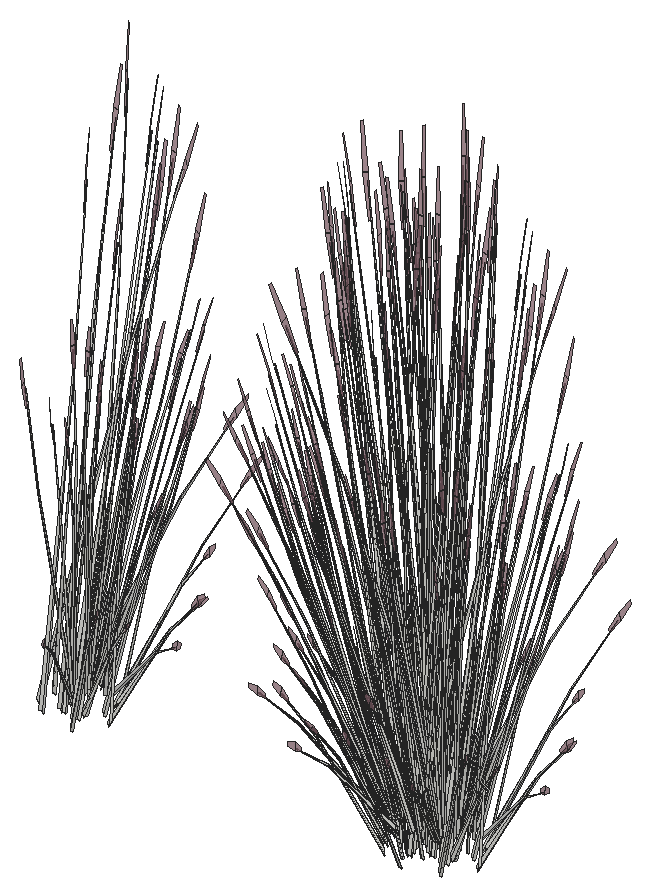
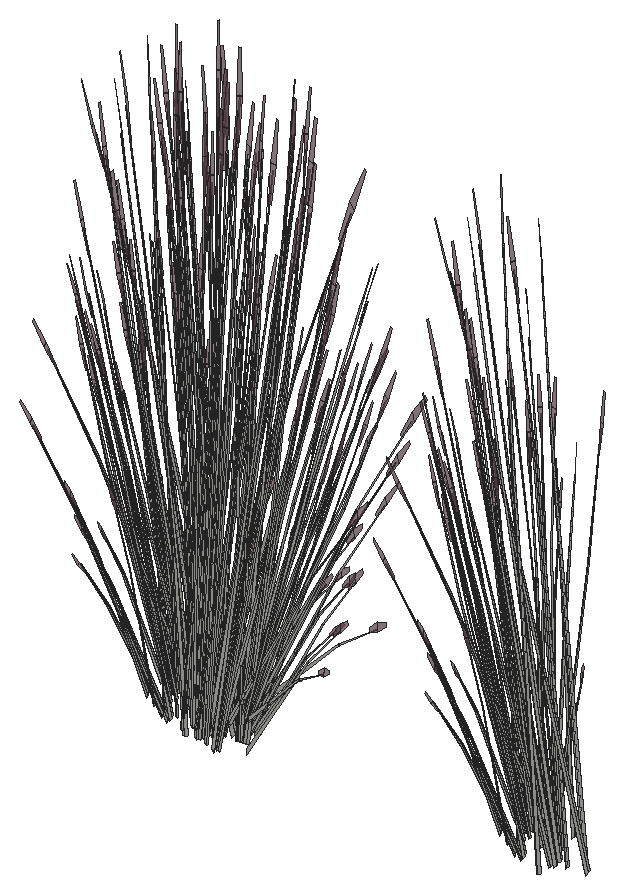
# SketchUp Ruby script. Lengths in inches.
U = 1.inch
M = Sketchup.active_model
def pt(a) = Geom::Point3d.new(a.map { |v| v * U })
def face(e, loops, mat)
  f = e.add_face(loops[0].map { |a| pt(a) })
  loops[1..].each { |l| e.add_face(l.map { |a| pt(a) }).erase! }
  f.material = f.back_material = mat if mat
  f
end
# faces: each face lists its corners as indices into pts; further lists are holes
def faces(e, pts, list, mat = nil) = list.each { |f| face(e, (f[0].is_a?(Array) ? f : [f]).map { |l| l.map { |i| pts[i] } }, mat) }
# xy, xz, yz: faces in a plane at the given z, y or x. An outline is a flat list of corners, or four numbers for a rectangle; further outlines are holes
def ring(l) = l.size == 4 ? [[l[0], l[1]], [l[2], l[1]], [l[2], l[3]], [l[0], l[3]]] : l.each_slice(2).to_a
def flat(e, list, mat, &to3) = list.each { |f| face(e, (f[0].is_a?(Array) ? f : [f]).map { |l| ring(l).map { |u, v| to3.(u, v) } }, mat) }
def xy(e, z, list, mat = nil) = flat(e, list, mat) { |x, y| [x, y, z] }
def xz(e, y, list, mat = nil) = flat(e, list, mat) { |x, z| [x, y, z] }
def yz(e, x, list, mat = nil) = flat(e, list, mat) { |y, z| [x, y, z] }
def lines(e, pts, list) = list.each { |a, b| e.add_line(pt(pts[a]), pt(pts[b])) }
# prism: a flat outline (further loops are holes) pulled along v
def prism(e, loops, v, mat = nil)
  f = face(e, loops, mat); d = Geom::Vector3d.new(v.map { |x| x * U })
  f.pushpull(f.normal.samedirection?(d) ? d.length : -d.length)
end
def box(e, o, s, mat = nil) = prism(e, [[o, [o[0] + s[0], o[1], o[2]], [o[0] + s[0], o[1] + s[1], o[2]], [o[0], o[1] + s[1], o[2]]]], [0, 0, s[2]], mat)
def at(x, y, z, deg = 0) = Geom::Transformation.translation(pt([x, y, z])) * Geom::Transformation.rotation(ORIGIN, Z_AXIS, deg.degrees)
def axes(o, x, y, z) = Geom::Transformation.new([*x, 0, *y, 0, *z, 0, *pt(o).to_a, 1])
def part(name) = M.definitions.add(name)
# library, detail: a bought-in or finely detailed component or shape, given as its bounding box
def library(name, o, s) = part(name).tap { |d| box(d.entities, o, s) }
def detail(e, o, s) = box(e.add_group.entities, o, s)
def put(e, d, t, mat = nil) = e.add_instance(d, t).tap { |i| i.material = mat if mat }
def group(e, t, mat = nil) = e.add_group.tap { |g| g.transformation = t; g.material = mat if mat }.entities
root = M.entities
M.materials.add("LightPink_Translucent").color = [144, 107, 117]
M.materials["LightPink_Translucent"].alpha = 0.75
c1 = part("blade")
p = [[2.15,0.21,22],[0,0.17,0],[0.09,0.45,0],[2.18,0.31,22],[2.29,0.31,22],[0.38,0.45,0],
  [2.48,0.24,33],[2.49,0.24,33],[2.48,0.22,33]]
faces(c1.entities,p,[[0,1,2,3],[4,5,2,3],[6,3,4,7],[8,0,3,6]])
c2 = part("seeds")
p = [[0.3,-0.1,1.38],[-0.01,-0.03,1.59],[-0.01,-0.03,0.03],[0.14,-0.07,-0.07],[0.29,-0.03,3],[0.15,0.01,3.11]]
faces(c2.entities,p,[[0,1,2,3],[1,0,4,5]],"LightPink_Translucent")
c3 = part("blade with seeds")
put(c3.entities,c1,at(0,0,0))
put(c3.entities,c2,axes([2.4,0.25,30.99],[1.5799,-0.05474,1.17369],[-0.12525,1.92788,0.29478],[-0.07173,-0.02425,1.56792]))
put(root,c3,axes([418.52,10.6,-2.125],[0.17368,0.19618,1.71376],[-0.80256,0.16516,0.13857],[-0.18139,-0.30799,0.73262]))
put(root,c3,axes([419.84,9.3,-1.28],[-0.11621,-0.08567,1.74944],[-0.77555,0.05431,-0.27667],[-0.12378,-0.20491,0.14031]))
put(root,c3,axes([421.64,10.3125,-3.41],[-0.21597,0.12368,1.43002],[-0.64681,-0.21647,-0.30754],[0.1199,-0.26922,0.61141]))
put(root,c3,axes([420.66,10.74,-1.02],[-0.36264,-0.49684,-0.71045],[0.74649,-0.27689,0.08574],[-0.0848,-0.24006,1.00501]))
put(root,c3,axes([418.3,10.08,-3.41],[-0.04601,0.19989,1.43002],[-0.67263,0.16733,-0.30754],[-0.15723,-0.25836,0.61141]))
put(root,c3,axes([420.03,9.64,-4.51],[-0.12744,0.02202,1.76342],[-0.70477,-0.24781,-0.26939],[0.01183,-0.2067,0.30037]))
put(root,c3,axes([385.75,11.23,-1.02],[0.01977,-0.56521,-0.71045],[0.83252,0.03796,0.08574],[0.08786,-0.23945,1.00501]))
put(root,c3,axes([422.17,11.23,-1.02],[0.01977,-0.56521,-0.71045],[0.83252,0.03796,0.08574],[0.08786,-0.23945,1.00501]))
put(root,c3,axes([386.91,10.35,-1.28],[-0.00733,-0.12161,1.74944],[-0.61946,-0.35147,-0.27667],[0.09577,-0.21306,0.14031]))
put(root,c3,axes([423.33,10.35,-1.28],[-0.00733,-0.12161,1.74944],[-0.61946,-0.35147,-0.27667],[0.09577,-0.21306,0.14031]))
put(root,c3,axes([420.73,10.32,-1.47],[0.22906,-0.4699,-0.35414],[0.66828,0.13705,0.4572],[-0.06128,-0.18919,0.87481]))
put(root,c3,axes([384.8125,10.94,-2.125],[-0.14147,0.21002,1.71376],[-0.59349,-0.43464,0.13857],[0.26773,-0.27089,0.73262]))
put(root,c3,axes([421.23,10.94,-2.125],[-0.14147,0.21002,1.71376],[-0.59349,-0.43464,0.13857],[0.26773,-0.27089,0.73262]))
put(root,c3,axes([423.16,9.91,-1.29],[-0.07716,0.04667,1.77383],[-0.75601,-0.15746,-0.16761],[-0.02737,-0.20368,0.31391]))
put(root,c3,axes([420.39,10.64,-1.32],[-0.7469,-0.15318,-0.51099],[0.25601,-0.52518,-0.3958],[-0.06849,-0.21144,0.97773]))
put(root,c3,axes([420.85,9.33,-3.23],[0.09747,0.35631,1.1486],[-0.54071,-0.19735,0.84392],[0.05818,-0.18244,0.25299]))
put(root,c3,axes([422,11.04,-1.32],[-0.54391,-0.41056,-0.51099],[0.57458,-0.35956,-0.3958],[0.08276,-0.2086,0.97773]))
put(root,c3,axes([419.05,9.02,-1.29],[-0.01417,0.07324,1.77383],[-0.6991,0.2658,-0.16761],[-0.20573,-0.13587,0.31391]))
put(root,c3,axes([418.9,10.31,-0.91],[0.84639,-0.15705,0.53763],[0.14689,0.61608,0.4433],[-0.19906,-0.18157,1.11249]))
put(root,c3,axes([420.81,10.43,-1.27],[0.74868,0.15974,0.48003],[-0.25601,0.52518,0.3958],[-0.04499,-0.20653,0.9933]))
put(root,c3,axes([421.02,10.62,-0.97],[-0.74352,0.28449,-0.1216],[-0.36538,-0.50492,-0.67495],[-0.0981,-0.21277,1.02557]))
put(root,c3,axes([422.57,11.26,-0.97],[-0.83505,-0.03027,-0.1216],[0.02282,-0.57322,-0.67495],[0.05801,-0.22077,1.02557]))
put(root,c3,axes([386.09,10.89,-1.47],[0.5141,-0.32171,-0.35414],[0.48666,0.36734,0.4572],[0.07405,-0.18664,0.87481]))
put(root,c3,axes([422.51,10.89,-1.47],[0.5141,-0.32171,-0.35414],[0.48666,0.36734,0.4572],[0.07405,-0.18664,0.87481]))
put(root,c3,axes([418.07,9.76,-3.23],[0.39634,0.21267,1.1486],[-0.57721,0.12784,0.84392],[-0.1235,-0.16344,0.25299]))
put(root,c3,axes([421.01,10.39,-1.27],[0.55987,-0.20767,0.0643],[0.27403,0.37869,0.50621],[-0.05407,-0.16693,0.77189]))
put(root,c3,axes([419.02,10.88,-1.02],[-0.64788,-0.29534,-0.71045],[0.46044,-0.51755,0.08574],[-0.23473,-0.17635,1.00501]))
put(root,c3,axes([418.8,10.49,-1.47],[-0.11735,-0.49217,-0.35414],[0.67083,-0.12996,0.4572],[-0.18018,-0.14104,0.87481]))
put(root,c3,axes([419.09,10.45,-1.27],[0.34533,-0.38816,0.0643],[0.49176,0.22599,0.50621],[-0.15898,-0.12445,0.77189]))
put(root,c3,axes([417.75,10.4,-4.51],[-0.0736,0.08049,1.76342],[-0.74378,0.17355,-0.26939],[-0.17968,-0.15788,0.30037]))
put(root,c3,axes([418.98,12.61,-3.9],[-0.31203,-0.62659,-0.69835],[0.89884,-0.22566,-0.18329],[-0.03449,-0.21218,1.54149]))
put(root,c3,axes([417.36,11.21,-2.125],[0.28223,0.10528,1.71376],[-0.58406,0.44165,0.13857],[-0.36402,-0.19924,0.73262]))
put(root,c3,axes([386.73,10.69,-4.51],[-0.11372,-0.04814,1.76342],[-0.29211,-0.53779,-0.26939],[0.19706,-0.14594,0.30037]))
put(root,c3,axes([423.15,10.69,-4.51],[-0.11372,-0.04814,1.76342],[-0.29211,-0.53779,-0.26939],[0.19706,-0.14594,0.30037]))
put(root,c3,axes([420.8,10.82,-0.95],[-0.22906,0.4699,0.35414],[-0.66828,-0.13705,-0.4572],[-0.06128,-0.18919,0.87481]))
put(root,c3,axes([418.72,10.9,-1.32],[-0.74975,0.14525,-0.51099],[-0.13115,-0.55007,-0.3958],[-0.20138,-0.15763,0.97773]))
put(root,c3,axes([386.09,11.01,-1.27],[0.54105,0.41691,0.48003],[-0.57458,0.35956,0.3958],[0.0998,-0.1956,0.9933]))
put(root,c3,axes([422.51,11.01,-1.27],[0.54105,0.41691,0.48003],[-0.57458,0.35956,0.3958],[0.0998,-0.1956,0.9933]))
put(root,c3,axes([419.25,10.41,-0.57],[-0.50709,0.58578,-0.13619],[-0.73436,-0.33748,-0.75594],[-0.25527,-0.1655,1.14864]))
put(root,c3,axes([386.29,11.05,-1.27],[0.62439,0.02847,0.0643],[-0.01712,0.42991,0.50621],[0.06534,-0.16468,0.77189]))
put(root,c3,axes([422.71,11.05,-1.27],[0.62439,0.02847,0.0643],[-0.01712,0.42991,0.50621],[0.06534,-0.16468,0.77189]))
put(root,c3,axes([422.24,11.35,-0.95],[-0.5141,0.32171,0.35414],[-0.48666,-0.36734,-0.4572],[0.07405,-0.18664,0.87481]))
put(root,c3,axes([386.73,12.21,-1.02],[0.39688,-0.48213,-0.71045],[0.69548,0.34264,0.08574],[0.23697,-0.17468,1.00501]))
put(root,c3,axes([423.15,12.21,-1.02],[0.39688,-0.48213,-0.71045],[0.69548,0.34264,0.08574],[0.23697,-0.17468,1.00501]))
put(root,c3,axes([418.86,10.81,-3.625],[-0.47504,-0.61229,0],[0.79476,-0.34146,-0.51607],[0.18101,-0.07777,1.63711]))
put(root,c3,axes([386.71,11.99,-1.32],[-0.19519,-0.55794,-0.51099],[0.73919,-0.0976,-0.3958],[0.21183,-0.14986,0.97773]))
put(root,c3,axes([423.13,11.99,-1.32],[-0.19519,-0.55794,-0.51099],[0.73919,-0.0976,-0.3958],[0.21183,-0.14986,0.97773]))
put(root,c3,axes([419.9,10.07,-3.87],[-0.52505,0.35054,-0.03893],[-0.48109,-0.38392,-0.17649],[-0.03387,-0.10878,0.58215]))
put(root,c3,axes([417.3,10.24,-1.28],[-0.16348,-0.00431,1.74944],[-0.52047,0.43131,-0.27667],[-0.2777,-0.08813,0.14031]))
put(root,c3,axes([387.06,12.39,-0.97],[-0.70283,-0.33692,-0.1216],[0.40491,-0.48793,-0.67495],[0.19857,-0.16961,1.02557]))
put(root,c3,axes([423.48,12.39,-0.97],[-0.70283,-0.33692,-0.1216],[0.40491,-0.48793,-0.67495],[0.19857,-0.16961,1.02557]))
put(root,c3,axes([420.57,14.22,-2.67],[0.65659,0.2464,1.51261],[-0.64324,0.53082,0.59816],[-0.28812,-0.31461,1.26806]))
put(root,c3,axes([419.2,10.89,-0.95],[0.11735,0.49217,0.35414],[-0.67083,0.12996,-0.4572],[-0.18018,-0.14104,0.87481]))
put(root,c3,axes([417.14,12.52,-3.98],[0,-0.61104,-0.49651],[0.85008,0,0],[0,-0.13917,1.57504]))
put(root,c3,axes([383.09,10.71,-3.98],[0.7111,-0.30552,-0.49651],[0.42504,0.54784,0],[0.16196,-0.06958,1.57504]))
put(root,c3,axes([419.5,10.71,-3.98],[0.7111,-0.30552,-0.49651],[0.42504,0.54784,0],[0.16196,-0.06958,1.57504]))
put(root,c3,axes([387.31,11.77,-3.41],[-0.27143,-0.0181,1.43002],[-0.27808,-0.48551,-0.30754],[0.33346,-0.13735,0.61141]))
put(root,c3,axes([423.72,11.77,-3.41],[-0.27143,-0.0181,1.43002],[-0.27808,-0.48551,-0.30754],[0.33346,-0.13735,0.61141]))
put(root,c3,axes([417.18,11.21,-0.91],[0.62747,-0.45094,0.53763],[0.54116,0.47889,0.4433],[-0.29439,-0.08318,1.11249]))
put(root,c3,axes([388.79,12.24,-1.29],[-0.09924,-0.00464,1.77383],[-0.4121,-0.49725,-0.16761],[0.1655,-0.1635,0.31391]))
put(root,c3,axes([425.21,12.24,-1.29],[-0.09924,-0.00464,1.77383],[-0.4121,-0.49725,-0.16761],[0.1655,-0.1635,0.31391]))
put(root,c3,axes([383.93,11.97,-3.94],[0.51177,-0.45928,-0.62353],[0.63575,0.41646,-0.16365],[0.20507,-0.11457,1.37633]))
put(root,c3,axes([420.35,11.97,-3.94],[0.51177,-0.45928,-0.62353],[0.63575,0.41646,-0.16365],[0.20507,-0.11457,1.37633]))
put(root,c3,axes([387.62,10.875,-3.23],[-0.25308,0.31105,1.1486],[-0.21753,-0.4179,0.84392],[0.20902,-0.10472,0.25299]))
put(root,c3,axes([424.04,10.875,-3.23],[-0.25308,0.31105,1.1486],[-0.21753,-0.4179,0.84392],[0.20902,-0.10472,0.25299]))
put(root,c3,axes([387.26,12.04,-1.47],[0.66138,-0.08733,-0.35414],[0.17464,0.49921,0.4572],[0.18953,-0.13408,0.87481]))
put(root,c3,axes([423.67,12.04,-1.47],[0.66138,-0.08733,-0.35414],[0.17464,0.49921,0.4572],[0.18953,-0.13408,0.87481]))
put(root,c3,axes([417.47,11.21,-1.27],[0.03826,-0.46465,0.0643],[0.57772,0.01274,0.50621],[-0.2213,-0.04862,0.77189]))
put(root,c3,axes([419.46,12.77,-3.79],[0.36864,-0.55059,-0.44739],[0.76598,0.26498,0.21531],[0,-0.12692,1.43643]))
put(root,c3,axes([417.25,11.36,-1.47],[-0.43232,-0.38257,-0.35414],[0.49364,-0.36215,0.4572],[-0.25081,-0.0551,0.87481]))
put(root,c3,axes([419.79,12.5,-3.33],[-0.08854,-0.69723,-0.29095],[0.92215,-0.04216,-0.50002],[0.16238,-0.09287,1.59708]))
put(root,c3,axes([417.51,12.54,-3.97],[0.53038,-0.38124,-0.30978],[0.53038,0.38124,0.30978],[0,-0.1228,1.38974]))
put(root,c3,axes([417.29,10.71,-3.87],[-0.21918,0.49894,-0.03893],[-0.6746,-0.15348,-0.17649],[-0.10242,-0.08161,0.58215]))
put(root,c3,axes([386.72,12.34,-0.95],[-0.66138,0.08733,0.35414],[-0.17464,-0.49921,-0.4572],[0.18953,-0.13408,0.87481]))
put(root,c3,axes([423.14,12.34,-0.95],[-0.66138,0.08733,0.35414],[-0.17464,-0.49921,-0.4572],[0.18953,-0.13408,0.87481]))
put(root,c3,axes([419.36,13.23,-3.33],[-0.85568,-0.29155,-0.29095],[0.41201,-0.61537,-0.50002],[-0.02689,-0.15109,1.59708]))
put(root,c3,axes([416.93,12.99,-3.625],[-0.95008,0,0],[0,-0.68292,-0.51607],[0,-0.15554,1.63711]))
put(root,c3,axes([417.09,11.76,-3.41],[0.14835,0.17012,1.43002],[-0.34183,0.46242,-0.30754],[-0.351,-0.11053,0.61141]))
put(root,c3,axes([419.67,10.95,-3.97],[0.70886,0.15119,-0.30978],[-0.17848,0.53243,0.30978],[0.1429,-0.0614,1.38974]))
put(root,c3,axes([417.7,11.61,-1.02],[-0.75952,-0.01471,-0.71045],[0.05101,-0.61953,0.08574],[-0.32177,-0.06538,1.00501]))
put(root,c3,axes([387.32,12.26,-1.27],[0.52161,0.25698,0.0643],[-0.30368,0.36595,0.50621],[0.16723,-0.11831,0.77189]))
put(root,c3,axes([423.73,12.26,-1.27],[0.52161,0.25698,0.0643],[-0.30368,0.36595,0.50621],[0.16723,-0.11831,0.77189]))
put(root,c3,axes([387.17,12.15,-1.27],[0.18844,0.56237,0.48003],[-0.73919,0.0976,0.3958],[0.21785,-0.13226,0.9933]))
put(root,c3,axes([423.59,12.15,-1.27],[0.18844,0.56237,0.48003],[-0.73919,0.0976,0.3958],[0.21785,-0.13226,0.9933]))
put(root,c3,axes([389.16,12.83,-1.28],[0.10543,-0.09307,1.74944],[-0.13495,-0.57092,-0.27667],[0.26455,-0.10825,0.14031]))
put(root,c3,axes([425.58,12.83,-1.28],[0.10543,-0.09307,1.74944],[-0.13495,-0.57092,-0.27667],[0.26455,-0.10825,0.14031]))
put(root,c3,axes([417.67,12.81,-3.67],[-0.70674,0.51372,0.30756],[-0.70717,-0.50832,-0.36492],[-0.02468,-0.14589,1.64885]))
put(root,c3,axes([416.67,10.6,-1.29],[0.05633,0.06098,1.77383],[-0.27155,0.54815,-0.16761],[-0.27501,0.00397,0.31391]))
put(root,c3,axes([419.91,13.04,-3.57],[0.8561,0.29616,0.24065],[-0.41201,0.61537,0.50002],[0,-0.14185,1.60543]))
put(root,c3,axes([419.58,13.875,-3.5625],[0.20138,-0.72405,-0.23429],[0.95485,0.12621,0.51271],[-0.16685,-0.09999,1.5644]))
put(root,c3,axes([417.45,11.74,-1.32],[-0.55171,0.40476,-0.51099],[-0.48318,-0.42758,-0.3958],[-0.28031,-0.06159,0.97773]))
put(root,c3,axes([417.86,11.56,-0.95],[0.43232,0.38257,0.35414],[-0.49364,0.36215,-0.4572],[-0.25081,-0.0551,0.87481]))
put(root,c3,axes([416.21,12.28,-3.23],[0.48508,-0.04372,1.1486],[-0.3077,0.38525,0.84392],[-0.23971,-0.05779,0.25299]))
put(root,c3,axes([419.64,12.63,-3.28],[-0.82508,0.03772,0.44739],[-0.07462,-0.62614,-0.21531],[0.14771,-0.06346,1.43643]))
put(root,c3,axes([417.74,11.32,-0.97],[-0.04068,0.62141,-0.1216],[-0.77029,-0.01698,-0.67495],[-0.29667,-0.04317,1.02557]))
put(root,c3,axes([417.51,13.09,-3.52],[0,0.61104,0.49651],[-0.85008,0,0],[0,-0.13917,1.57504]))
put(root,c3,axes([387.09,13.7,-0.97],[-0.38229,-0.5533,-0.1216],[0.6785,-0.2719,-0.67495],[0.28593,-0.073,1.02557]))
put(root,c3,axes([423.51,13.7,-0.97],[-0.38229,-0.5533,-0.1216],[0.6785,-0.2719,-0.67495],[0.28593,-0.073,1.02557]))
put(root,c3,axes([387.05,13.22,-1.32],[0.20584,-0.55581,-0.51099],[0.70573,0.19051,-0.3958],[0.28414,-0.05097,0.97773]))
put(root,c3,axes([423.47,13.22,-1.32],[0.20584,-0.55581,-0.51099],[0.70573,0.19051,-0.3958],[0.28414,-0.05097,0.97773]))
put(root,c3,axes([385.9375,10.96,-3.625],[0.47504,-0.61229,0],[0.79476,0.34146,-0.51607],[0.18101,0.07777,1.63711]))
put(root,c3,axes([422.36,10.96,-3.625],[0.47504,-0.61229,0],[0.79476,0.34146,-0.51607],[0.18101,0.07777,1.63711]))
put(root,c3,axes([416.76,12.17,-2.125],[0.31515,-0.01384,1.71376],[-0.20907,0.5998,0.13857],[-0.44912,-0.0371,0.73262]))
put(root,c3,axes([419.51,13.58,-3.79],[-0.45644,-0.51287,-0.44739],[0.69137,-0.36116,0.21531],[-0.14771,-0.06346,1.43643]))
put(root,c3,axes([419.61,12.86,-3.64],[0.33034,0.68327,0.45755],[-0.94388,0.2376,0.17955],[0.01154,-0.12555,1.58856]))
put(root,c3,axes([387.81,13.38,-4.02],[-0.48937,0.07333,1.41583],[-0.07789,-0.58369,0.08104],[0.34275,-0.08835,0.80566]))
put(root,c3,axes([424.23,13.38,-4.02],[-0.48937,0.07333,1.41583],[-0.07789,-0.58369,0.08104],[0.34275,-0.08835,0.80566]))
put(root,c3,axes([388.7,12.86,-3.74],[-0.47106,-0.39072,-0.06488],[0.51591,-0.35801,-0.29416],[0.14618,-0.02521,0.97024]))
put(root,c3,axes([425.12,12.86,-3.74],[-0.47106,-0.39072,-0.06488],[0.51591,-0.35801,-0.29416],[0.14618,-0.02521,0.97024]))
put(root,c3,axes([419.44,13.4,-3.28],[-0.36864,0.55059,0.44739],[-0.76598,-0.26498,-0.21531],[0,-0.12692,1.43643]))
put(root,c3,axes([420.8,12.92,-3.79],[0,-0.70701,0],[0.95008,0,0],[0,0,1.79456]))
put(root,c3,axes([385.53,11.28,-3.52],[-0.7111,-0.30552,0.49651],[0.42504,-0.54784,0],[0.16196,0.06958,1.57504]))
put(root,c3,axes([421.95,11.28,-3.52],[-0.7111,-0.30552,0.49651],[0.42504,-0.54784,0],[0.16196,0.06958,1.57504]))
put(root,c3,axes([386.92,13.43,-1.02],[0.66765,-0.26986,-0.71045],[0.37208,0.55551,0.08574],[0.32259,-0.0631,1.00501]))
put(root,c3,axes([423.34,13.43,-1.02],[0.66765,-0.26986,-0.71045],[0.37208,0.55551,0.08574],[0.32259,-0.0631,1.00501]))
put(root,c3,axes([419.1,13.78,-3.94],[-0.79037,-0.10018,-0.62353],[0.16679,-0.61794,-0.16365],[-0.23587,-0.07488,1.37633]))
put(root,c3,axes([420.35,12.47,-3.64],[-0.62999,0.55453,0.45755],[-0.74845,-0.4895,0.17955],[0.15188,-0.05534,1.58856]))
put(root,c3,axes([421.03,13.46,-3.7],[-0.70674,-0.52593,-0.06131],[0.70717,-0.52625,0],[-0.02468,-0.01837,1.75571]))
put(root,c3,axes([419.25,11.56,-3.53],[-0.21949,0.60727,0.17642],[-0.8032,-0.17185,0.35086],[0.13875,-0.00296,1.60407]))
put(root,c3,axes([386.82,13.53,-0.95],[-0.63144,-0.17046,0.35414],[0.18417,-0.49731,-0.4572],[0.25423,-0.0456,0.87481]))
put(root,c3,axes([423.24,13.53,-0.95],[-0.63144,-0.17046,0.35414],[0.18417,-0.49731,-0.4572],[0.25423,-0.0456,0.87481]))
put(root,c3,axes([416.63,12.625,-1.27],[0.21466,-0.55714,0.48003],[0.70573,0.19051,0.3958],[-0.27753,0.03348,0.9933]))
put(root,c3,axes([382.5,12.05,-4.41],[-0.74787,0.24464,1.28929],[-0.23804,-0.70192,0.50096],[0.45924,0.01168,1.46642]))
put(root,c3,axes([418.92,12.05,-4.41],[-0.74787,0.24464,1.28929],[-0.23804,-0.70192,0.50096],[0.45924,0.01168,1.46642]))
put(root,c3,axes([384.51,12.23,-3.38],[0.14658,-0.54532,0.1448],[0.71613,0.09466,-0.41347],[0.13033,0.05599,1.26744]))
put(root,c3,axes([420.93,12.23,-3.38],[0.14658,-0.54532,0.1448],[0.71613,0.09466,-0.41347],[0.13033,0.05599,1.26744]))
put(root,c3,axes([416.58,12.48,-1.27],[-0.27906,-0.41663,0.0643],[0.50888,-0.20393,0.50621],[-0.22432,0.04024,0.77189]))
put(root,c3,axes([419.69,13.53,-3.64],[0.96033,0.12874,0.45755],[-0.19544,0.7271,0.17955],[-0.14034,-0.07021,1.58856]))
put(root,c3,axes([388.34,13,-4.51],[-0.03971,-0.09277,1.76342],[0.27541,-0.54264,-0.26939],[0.27782,-0.00781,0.30037]))
put(root,c3,axes([424.76,13,-4.51],[-0.03971,-0.09277,1.76342],[0.27541,-0.54264,-0.26939],[0.27782,-0.00781,0.30037]))
put(root,c3,axes([416.5625,12.91,-4.51],[0.01927,0.0963,1.76342],[-0.38846,0.5029,-0.26939],[-0.27592,-0.02535,0.30037]))
put(root,c3,axes([420.62,12.375,-3.28],[-0.45644,-0.51287,0.44739],[0.69137,-0.36116,-0.21531],[0.14771,0.06346,1.43643]))
put(root,c3,axes([418.26,14.72,-3.97],[-0.17848,-0.53243,-0.30978],[0.70886,-0.15119,0.30978],[-0.1429,-0.0614,1.38974]))
put(root,c3,axes([419.17,14.6875,-3.53],[0.81646,-0.16218,0.17642],[0.20161,0.60355,0.35086],[-0.07282,-0.08794,1.60407]))
put(root,c3,axes([384.4375,12.41,-3.33],[0.76714,-0.40567,-0.29095],[0.51013,0.57321,-0.50002],[0.18927,0.05821,1.59708]))
put(root,c3,axes([420.86,12.41,-3.33],[0.76714,-0.40567,-0.29095],[0.51013,0.57321,-0.50002],[0.18927,0.05821,1.59708]))
put(root,c3,axes([387.49,13.48,-1.47],[0.63144,0.17046,-0.35414],[-0.18417,0.49731,0.4572],[0.25423,-0.0456,0.87481]))
put(root,c3,axes([423.91,13.48,-1.47],[0.63144,0.17046,-0.35414],[-0.18417,0.49731,0.4572],[0.25423,-0.0456,0.87481]))
put(root,c3,axes([418.07,14.95,-3.98],[-0.7111,-0.30552,-0.49651],[0.42504,-0.54784,0],[-0.16196,-0.06958,1.57504]))
put(root,c3,axes([386.37,11.33,-3.98],[0.7111,0.30552,-0.49651],[-0.42504,0.54784,0],[0.16196,0.06958,1.57504]))
put(root,c3,axes([422.79,11.33,-3.98],[0.7111,0.30552,-0.49651],[-0.42504,0.54784,0],[0.16196,0.06958,1.57504]))
put(root,c3,axes([416.48,12.6875,-1.47],[-0.63144,-0.17046,-0.35414],[0.18417,-0.49731,0.4572],[-0.25423,0.0456,0.87481]))
put(root,c3,axes([421.44,13.07,-3.79],[0.85008,0,0],[0,0.63259,0],[0,0,1.78407]))
put(root,c3,axes([420,13.87,-3.33],[-0.76714,0.40567,-0.29095],[-0.51013,-0.57321,-0.50002],[-0.18927,-0.05821,1.59708]))
put(root,c3,axes([421.68,11.59,-3.53],[-0.81646,0.16218,0.17642],[-0.20161,-0.60355,0.35086],[0.07282,0.08794,1.60407]))
put(root,c3,axes([385.77,12.86,-2.125],[-0.31515,0.01384,1.71376],[0.20907,-0.5998,0.13857],[0.44912,0.0371,0.73262]))
put(root,c3,axes([422.18,12.86,-2.125],[-0.31515,0.01384,1.71376],[0.20907,-0.5998,0.13857],[0.44912,0.0371,0.73262]))
put(root,c3,axes([386.17,11.56,-3.97],[0.17848,0.53243,-0.30978],[-0.70886,0.15119,0.30978],[0.1429,0.0614,1.38974]))
put(root,c3,axes([422.59,11.56,-3.97],[0.17848,0.53243,-0.30978],[-0.70886,0.15119,0.30978],[0.1429,0.0614,1.38974]))
put(root,c3,axes([387.39,13.6875,-1.27],[0.27906,0.41663,0.0643],[-0.50888,0.20393,0.50621],[0.22432,-0.04024,0.77189]))
put(root,c3,axes([423.8125,13.6875,-1.27],[0.27906,0.41663,0.0643],[-0.50888,0.20393,0.50621],[0.22432,-0.04024,0.77189]))
put(root,c3,axes([421.17,12.75,-3.62],[-0.96033,-0.12874,0.49198],[0.19544,-0.7271,0.19306],[0.14034,0.07021,1.70813]))
put(root,c3,axes([387.34,13.54,-1.27],[-0.21466,0.55714,0.48003],[-0.70573,-0.19051,0.3958],[0.27753,-0.03348,0.9933]))
put(root,c3,axes([423.76,13.54,-1.27],[-0.21466,0.55714,0.48003],[-0.70573,-0.19051,0.3958],[0.27753,-0.03348,0.9933]))
put(root,c3,axes([420.4,14.55,-3.8],[-0.24791,-0.5268,0],[0.70791,-0.18448,0],[0,0,1.54371]))
put(root,c3,axes([419.93,14.05,-3.38],[-0.14658,0.54532,0.1448],[-0.71613,-0.09466,-0.41347],[-0.13033,-0.05599,1.26744]))
put(root,c3,axes([417.15,12.63,-0.95],[0.63144,0.17046,0.35414],[-0.18417,0.49731,-0.4572],[-0.25423,0.0456,0.87481]))
put(root,c3,axes([384.91,14.47,-3.82],[0.79769,-0.20732,-0.19198],[0.2803,0.59721,0.00008],[0.08805,-0.02292,1.73897]))
put(root,c3,axes([421.33,14.47,-3.82],[0.79769,-0.20732,-0.19198],[0.2803,0.59721,0.00008],[0.08805,-0.02292,1.73897]))
put(root,c3,axes([421.6,14.72,-3.53],[0.21949,-0.60727,0.17642],[0.8032,0.17185,0.35086],[-0.13875,0.00296,1.60407]))
put(root,c3,axes([421.42,13.34,-3.79],[0.53038,0.39469,0],[-0.53038,0.39469,0],[0,0,1.69266]))
put(root,c3,axes([418.41,12.6,-2.66],[0.21597,-0.08839,1.77064],[0.07448,0.61717,0.13857],[-0.4678,0.08189,0.63284]))
put(root,c3,axes([422.86,13.17,-3.53],[-0.59697,-0.44509,0.17642],[0.60159,-0.4317,0.35086],[-0.06593,0.0909,1.60407]))
put(root,c3,axes([385.33,12.5,-3.94],[0.79037,0.10018,-0.62353],[-0.16679,0.61794,-0.16365],[0.23587,0.07488,1.37633]))
put(root,c3,axes([421.75,12.5,-3.94],[0.79037,0.10018,-0.62353],[-0.16679,0.61794,-0.16365],[0.23587,0.07488,1.37633]))
put(root,c3,axes([388.83,13.58,-3.23],[-0.46945,0.10088,1.1486],[0.22097,-0.4169,0.84392],[0.24904,0.02853,0.25299]))
put(root,c3,axes([425.24,13.58,-3.23],[-0.46945,0.10088,1.1486],[0.22097,-0.4169,0.84392],[0.24904,0.02853,0.25299]))
put(root,c3,axes([420.23,14.78,-3.8],[-0.76598,-0.27433,0],[0.36864,-0.57001,0],[0,0,1.62707]))
put(root,c3,axes([420.86,14.05,-3.54],[-0.74193,-0.49181,-0.25192],[0.6243,-0.55226,0.5513],[-0.19979,0.05753,1.68216]))
put(root,c3,axes([418.91,15,-3.52],[0.7111,0.30552,0.49651],[-0.42504,0.54784,0],[-0.16196,-0.06958,1.57504]))
put(root,c3,axes([421.41,12.88,-3.28],[0.36864,-0.55059,0.44739],[0.76598,0.26498,-0.21531],[0,0.12692,1.43643]))
put(root,c3,axes([388.61,15.34,-1.29],[-0.0687,-0.05349,1.77383],[0.15029,-0.57341,-0.16761],[0.27062,-0.03664,0.31391]))
put(root,c3,axes([425.03,15.34,-1.29],[-0.0687,-0.05349,1.77383],[0.15029,-0.57341,-0.16761],[0.27062,-0.03664,0.31391]))
put(root,c3,axes([416.09,13.02,-1.28],[-0.12407,0.07933,1.74944],[0.01055,0.57963,-0.27667],[-0.2844,0.07538,0.14031]))
put(root,c3,axes([421.27,13.2,-3.71],[0,0.70667,-0.05637],[-0.95008,0,0],[0,0.02221,1.79368]))
put(root,c3,axes([416.92,12.94,-1.32],[-0.20584,0.55581,-0.51099],[-0.70573,-0.19051,-0.3958],[-0.28414,0.05097,0.97773]))
put(root,c3,axes([416.88,12.46,-0.97],[0.38229,0.5533,-0.1216],[-0.6785,0.2719,-0.67495],[-0.28593,0.073,1.02557]))
put(root,c3,axes([384.92,12.7,-3.79],[0.45644,0.51287,-0.44739],[-0.69137,0.36116,0.21531],[0.14771,0.06346,1.43643]))
put(root,c3,axes([421.34,12.7,-3.79],[0.45644,0.51287,-0.44739],[-0.69137,0.36116,0.21531],[0.14771,0.06346,1.43643]))
put(root,c3,axes([388.01,14.87,-2.07],[-0.14542,-0.51365,-0.03492],[0.68734,-0.11809,-0.15832],[0.14353,0.03256,0.52218]))
put(root,c3,axes([424.43,14.87,-2.07],[-0.14542,-0.51365,-0.03492],[0.68734,-0.11809,-0.15832],[0.14353,0.03256,0.52218]))
put(root,c3,axes([418.5,15.32,-3.625],[-0.47504,0.61229,0],[-0.79476,-0.34146,-0.51607],[-0.18101,-0.07777,1.63711]))
put(root,c3,axes([386.23,14.85,-0.97],[0.04068,-0.62141,-0.1216],[0.77029,0.01698,-0.67495],[0.29667,0.04317,1.02557]))
put(root,c3,axes([422.65,14.85,-0.97],[0.04068,-0.62141,-0.1216],[0.77029,0.01698,-0.67495],[0.29667,0.04317,1.02557]))
put(root,c3,axes([423.35,13.19,-3.52],[0,-0.61104,0.49651],[0.85008,0,0],[0,0.13917,1.57504]))
put(root,c3,axes([421.22,13.65,-3.28],[0.82508,-0.03772,0.44739],[0.07462,0.62614,-0.21531],[-0.14771,0.06346,1.43643]))
put(root,c3,axes([421.73,13.01,-3.38],[0.70791,-0.1782,0.1448],[0.24791,0.50885,-0.41347],[0,0.11199,1.26744]))
put(root,c3,axes([386.11,14.61,-0.95],[-0.43232,-0.38257,0.35414],[0.49364,-0.36215,-0.4572],[0.25081,0.0551,0.87481]))
put(root,c3,axes([422.53,14.61,-0.95],[-0.43232,-0.38257,0.35414],[0.49364,-0.36215,-0.4572],[0.25081,0.0551,0.87481]))
put(root,c3,axes([420.49,13.95,-3.79],[-0.82508,0.03772,-0.44739],[-0.07462,-0.62614,0.21531],[-0.14771,0.06346,1.43643]))
put(root,c3,axes([387.95,14.25,-3.41],[-0.18299,-0.15028,1.43002],[0.23809,-0.49714,-0.30754],[0.37023,0.06735,0.61141]))
put(root,c3,axes([424.36,14.25,-3.41],[-0.18299,-0.15028,1.43002],[0.23809,-0.49714,-0.30754],[0.37023,0.06735,0.61141]))
